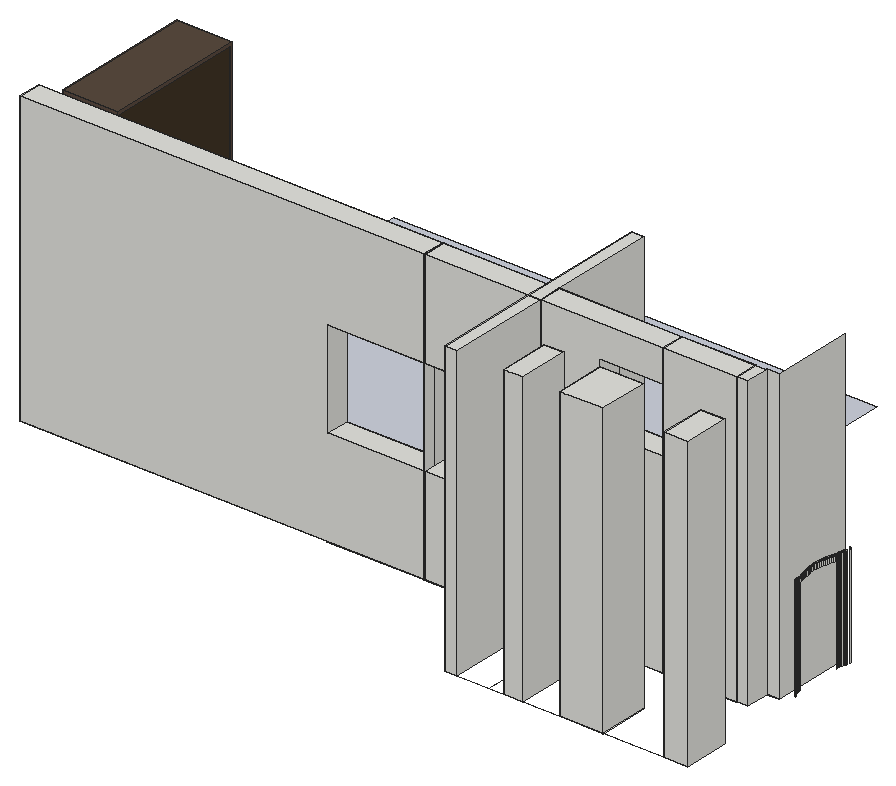
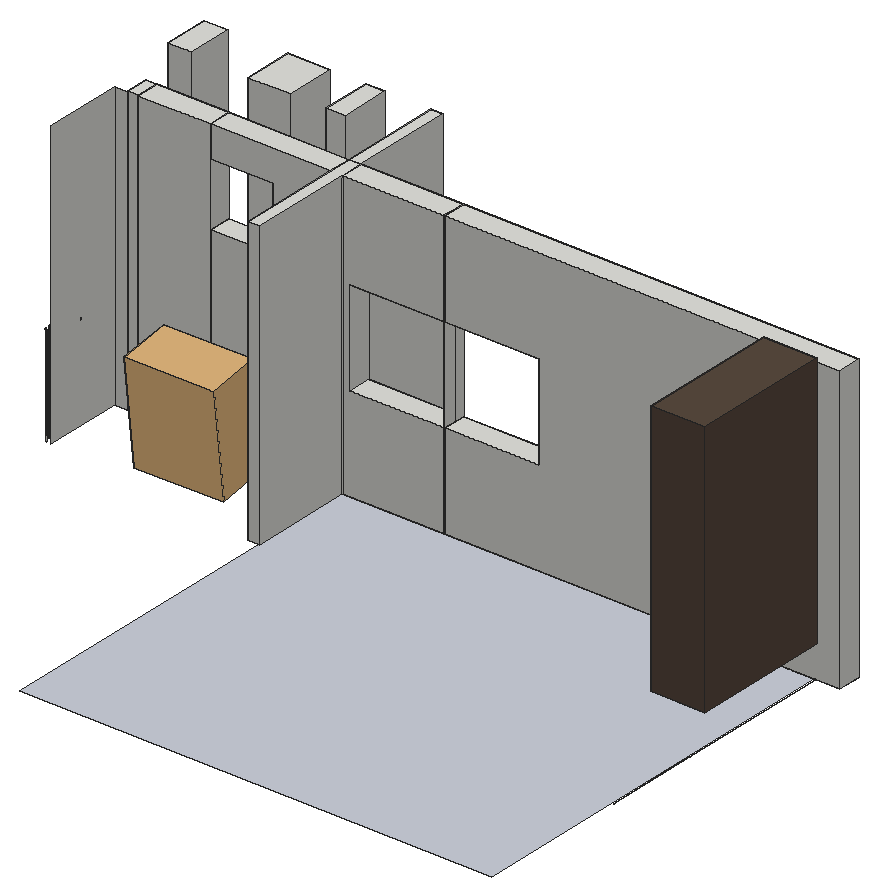
# SketchUp Ruby script. Lengths in inches.
U = 1.inch
M = Sketchup.active_model
def pt(a) = Geom::Point3d.new(a.map { |v| v * U })
def face(e, loops, mat)
  f = e.add_face(loops[0].map { |a| pt(a) })
  loops[1..].each { |l| e.add_face(l.map { |a| pt(a) }).erase! }
  f.material = f.back_material = mat if mat
  f
end
# faces: each face lists its corners as indices into pts; further lists are holes
def faces(e, pts, list, mat = nil) = list.each { |f| face(e, (f[0].is_a?(Array) ? f : [f]).map { |l| l.map { |i| pts[i] } }, mat) }
# xy, xz, yz: faces in a plane at the given z, y or x. An outline is a flat list of corners, or four numbers for a rectangle; further outlines are holes
def ring(l) = l.size == 4 ? [[l[0], l[1]], [l[2], l[1]], [l[2], l[3]], [l[0], l[3]]] : l.each_slice(2).to_a
def flat(e, list, mat, &to3) = list.each { |f| face(e, (f[0].is_a?(Array) ? f : [f]).map { |l| ring(l).map { |u, v| to3.(u, v) } }, mat) }
def xy(e, z, list, mat = nil) = flat(e, list, mat) { |x, y| [x, y, z] }
def xz(e, y, list, mat = nil) = flat(e, list, mat) { |x, z| [x, y, z] }
def yz(e, x, list, mat = nil) = flat(e, list, mat) { |y, z| [x, y, z] }
def lines(e, pts, list) = list.each { |a, b| e.add_line(pt(pts[a]), pt(pts[b])) }
# prism: a flat outline (further loops are holes) pulled along v
def prism(e, loops, v, mat = nil)
  f = face(e, loops, mat); d = Geom::Vector3d.new(v.map { |x| x * U })
  f.pushpull(f.normal.samedirection?(d) ? d.length : -d.length)
end
def box(e, o, s, mat = nil) = prism(e, [[o, [o[0] + s[0], o[1], o[2]], [o[0] + s[0], o[1] + s[1], o[2]], [o[0], o[1] + s[1], o[2]]]], [0, 0, s[2]], mat)
def at(x, y, z, deg = 0) = Geom::Transformation.translation(pt([x, y, z])) * Geom::Transformation.rotation(ORIGIN, Z_AXIS, deg.degrees)
def axes(o, x, y, z) = Geom::Transformation.new([*x, 0, *y, 0, *z, 0, *pt(o).to_a, 1])
def part(name) = M.definitions.add(name)
# library, detail: a bought-in or finely detailed component or shape, given as its bounding box
def library(name, o, s) = part(name).tap { |d| box(d.entities, o, s) }
def detail(e, o, s) = box(e.add_group.entities, o, s)
def put(e, d, t, mat = nil) = e.add_instance(d, t).tap { |i| i.material = mat if mat }
def group(e, t, mat = nil) = e.add_group.tap { |g| g.transformation = t; g.material = mat if mat }.entities
root = M.entities
M.materials.add("[Color A02]").color = [65, 53, 38]
M.materials.add("[Marble Carrara Floor Tile]").color = [204, 208, 219]
M.materials.add("[Wood Veneer 01]").color = [89, 74, 63]
c1 = library("Group\#73",[0,0,0],[33.36,19.5,40.28])
c2 = part("Component\#1")
xy(c2.entities,0,[[0,0,0,29.53,70.87,29.53,70.87,0,69.88,0,69.88,0.98,0.98,0.98,0.98,0]],"[Wood Veneer 01]")
xy(c2.entities,77.76,[[0.98,0,69.88,0.98]])
xy(c2.entities,78.74,[[0,0,70.87,29.53]],"[Wood Veneer 01]")
xz(c2.entities,0,[[0,0,0.98,0,0.98,77.76,69.88,77.76,69.88,0,70.87,0,70.87,78.74,0,78.74]],"[Wood Veneer 01]")
xz(c2.entities,0.98,[[0.98,0.98,69.88,77.76]])
xz(c2.entities,0.98,[[0.98,0,69.88,0.98]],"[Wood Veneer 01]")
xz(c2.entities,29.53,[[0,0,70.87,78.74]],"[Wood Veneer 01]")
yz(c2.entities,0,[[0,0,29.53,78.74]],"[Wood Veneer 01]")
yz(c2.entities,0.98,[[0,0,0.98,0.98],[0,0.98,0.98,77.76]],"[Wood Veneer 01]")
yz(c2.entities,69.88,[[0,0,0.98,0.98],[0,0.98,0.98,77.76]],"[Wood Veneer 01]")
yz(c2.entities,70.87,[[0,0,29.53,78.74]],"[Wood Veneer 01]")
xy(root,0,[[283.6875,0,299.97,0.09],[299.73,0.09,299.97,18.91],[166.56,38.625,202.24,38.86],[202.24,38.625,202.56,38.86],[202.56,38.625,238.24,38.86],
  [282.63,38.625,291.08,38.86],[291.08,38.625,318.375,38.86],[318.375,38.625,318.63,38.86],[267.52,38.86,291.08,47.625],[291.08,38.86,318.375,47.625],
  [318.375,38.86,318.63,47.625],[62.1,45.23,241,45.23,241,47.86,83.3,47.86,83.3,47.83,62.1,47.83],[245.5,47.625,291.08,47.86],[291.08,47.625,318.375,47.86],[318.375,47.625,322.5,47.86],
  [322.5,47.625,327,47.86],[61.56,47.83,62.1,47.86],[62.1,47.83,72.0625,47.86],[61.5,47.86,61.56,107.65],[61.5,107.65,61.56,107.65,61.56,113,61.53,113,61.53,143.65,61.5,143.65]])
xy(root,0,[[62.1,47.86,241,200.36]],"[Marble Carrara Floor Tile]")
xz(root,47.86,[[322.5,0,327,108]])
yz(root,327,[[47.86,0,78.05,108]])
yz(root,328.72,[[54.53,0,54.73,37.7],[54.73,0,54.93,37.7],[72.76,0,72.96,37.7],[72.96,0,73.15,37.7],[54.53,37.7,54.73,37.8],
  [54.73,37.7,54.93,37.8],[72.76,37.7,72.96,37.8],[72.96,37.7,73.15,37.8]])
p = [[329.87,52.03,0],[329.87,52.03,37.7],[329.75,52.0625,37.7],[329.75,52.0625,0],[329.63,52.11,0],[329.63,52.11,37.7],
  [329.51,52.16,37.7],[329.51,52.16,0],[329.4,52.23,0],[329.4,52.23,37.7],[329.3,52.31,37.7],[329.3,52.31,0],
  [329.21,52.4,37.7],[329.21,52.4,0],[329.13,52.49,37.7],[329.13,52.49,0],[329.06,52.6,37.7],[329.06,52.6,0],
  [329,52.71,37.7],[329,52.71,0],[328.95,52.83,37.7],[328.95,52.83,0],[328.91,52.96,37.7],[328.91,52.96,0],
  [328.875,53.15,37.7],[328.875,53.15,0],[328.84,53.35,37.7],[328.84,53.35,0],[328.81,53.54,37.7],[328.81,53.54,0],
  [328.78,53.74,37.7],[328.78,53.74,0],[328.76,53.9375,37.7],[328.76,53.9375,0],[328.74,54.14,37.7],[328.74,54.14,0],
  [328.73,54.33,37.7],[328.73,54.33,0],[328.72,54.53,37.7],[328.72,54.53,0],[328.72,54.93,0],[328.72,54.93,37.7],
  [328.73,55.13,37.7],[328.73,55.13,0],[328.74,55.33,37.7],[328.74,55.33,35.76],[328.74,55.33,0],[328.74,72.36,35.76],
  [328.74,72.36,37.7],[328.73,72.56,37.7],[328.73,72.56,0],[328.74,72.36,0],[328.72,72.76,37.7],[328.72,72.76,0],
  [328.72,73.15,0],[328.72,73.15,37.7],[328.73,73.35,37.7],[328.73,73.35,0],[328.74,73.55,37.7],[328.74,73.55,0],
  [328.76,73.75,37.7],[328.76,73.75,0],[328.78,73.95,37.7],[328.78,73.95,0],[328.81,74.14,37.7],[328.81,74.14,0],
  [328.84,74.34,37.7],[328.84,74.34,0],[328.875,74.53,37.7],[328.875,74.53,0],[328.91,74.73,37.7],[328.91,74.73,0],
  [328.95,74.85,37.7],[328.95,74.85,0],[329,74.97,37.7],[329,74.97,0],[329.06,75.08,37.7],[329.06,75.08,0],
  [329.13,75.19,37.7],[329.13,75.19,0],[329.21,75.29,37.7],[329.21,75.29,0],[329.3,75.38,37.7],[329.3,75.38,0],
  [329.4,75.46,37.7],[329.4,75.46,0],[329.51,75.52,37.7],[329.51,75.52,0],[329.63,75.58,37.7],[329.63,75.58,0],
  [329.75,75.625,37.7],[329.75,75.625,0],[329.87,75.65,37.7],[329.87,75.65,0],[329.75,77.3125,0],[329.75,77.3125,37.7],
  [329.63,77.36,37.7],[329.63,77.36,0],[329.87,77.28,0],[329.87,77.28,37.7],[329.51,77.41,0],[329.51,77.41,37.7],
  [329.4,77.48,37.7],[329.4,77.48,0],[329.3,77.56,37.7],[329.3,77.56,0],[329.21,77.65,0],[329.21,77.65,37.7],
  [329.13,77.74,37.7],[329.13,77.74,0],[328.52,56.02,37.7],[328.52,56.02,35.76],[328.31,56.71,37.7],[328.31,56.71,35.76],
  [328.12,57.41,37.7],[328.12,57.41,35.76],[327.94,58.12,37.7],[327.94,58.12,35.76],[327.78,58.82,37.7],[327.78,58.82,35.76],
  [327.625,59.53,37.7],[327.625,59.53,35.76],[327.49,60.25,37.7],[327.49,60.25,35.76],[327.36,60.96,37.7],[327.36,60.96,35.76],
  [327.25,61.68,37.7],[327.25,61.68,35.76],[327.15,62.4,37.7],[327.15,62.4,35.76],[327.07,63.12,37.7],[327.07,63.12,35.76],
  [327,63.84,37.7],[327,63.84,35.76],[327.07,64.57,37.7],[327.07,64.57,35.76],[327.15,65.29,37.7],[327.15,65.29,35.76],
  [327.25,66.01,37.7],[327.25,66.01,35.76],[327.36,66.72,37.7],[327.36,66.72,35.76],[327.49,67.4375,37.7],[327.49,67.4375,35.76],
  [327.625,68.15,37.7],[327.625,68.15,35.76],[327.78,68.86,37.7],[327.78,68.86,35.76],[327.94,69.57,37.7],[327.94,69.57,35.76],
  [328.12,70.27,37.7],[328.12,70.27,35.76],[328.31,70.97,37.7],[328.31,70.97,35.76],[328.52,71.67,37.7],[328.52,71.67,35.76],
  [329.875,52.04,37.8],[329.75,52.07,37.8],[329.63,52.11,37.8],[329.51,52.16,37.8],[329.4,52.23,37.8],[329.3,52.31,37.8],
  [329.21,52.4,37.8],[329.13,52.5,37.8],[329.06,52.6,37.8],[329,52.72,37.8],[328.95,52.84,37.8],[328.92,52.96,37.8],
  [328.875,53.15,37.8],[328.84,53.35,37.8],[328.81,53.54,37.8],[328.78,53.74,37.8],[328.76,53.9375,37.8],[328.74,54.14,37.8],
  [328.73,54.33,37.8],[328.72,54.53,37.8],[328.72,54.93,37.8],[328.73,55.13,37.8],[328.74,55.33,37.8],[328.52,56.02,37.8],
  [328.32,56.72,37.8],[328.125,57.42,37.8],[327.95,58.12,37.8],[327.78,58.83,37.8],[327.63,59.54,37.8],[327.49,60.25,37.8],
  [327.37,60.96,37.8],[327.25,61.68,37.8],[327.16,62.4,37.8],[327.07,63.12,37.8],[327,63.84,37.8],[327.07,64.57,37.8],
  [327.16,65.29,37.8],[327.25,66.01,37.8],[327.37,66.72,37.8],[327.49,67.4375,37.8],[327.63,68.15,37.8],[327.78,68.86,37.8],
  [327.95,69.57,37.8],[328.125,70.27,37.8],[328.32,70.97,37.8],[328.52,71.67,37.8],[328.74,72.36,37.8],[328.73,72.56,37.8],
  [328.72,72.76,37.8],[328.72,73.15,37.8],[328.73,73.35,37.8],[328.74,73.55,37.8],[328.76,73.75,37.8],[328.78,73.95,37.8],
  [328.81,74.14,37.8],[328.84,74.34,37.8],[328.875,74.53,37.8],[328.92,74.73,37.8],[328.95,74.85,37.8],[329,74.97,37.8],
  [329.06,75.08,37.8],[329.13,75.1875,37.8],[329.21,75.29,37.8],[329.3,75.375,37.8],[329.4,75.45,37.8],[329.51,75.52,37.8],
  [329.63,75.58,37.8],[329.75,75.62,37.8],[329.875,75.65,37.8],[329.75,77.32,37.8],[329.63,77.36,37.8],[329.875,77.29,37.8],
  [329.51,77.41,37.8],[329.4,77.48,37.8],[329.3,77.56,37.8],[329.21,77.65,37.8],[329.875,52.05,37.89],[329.75,52.08,37.89],
  [329.63,52.12,37.89],[329.52,52.17,37.89],[329.41,52.24,37.89],[329.3125,52.32,37.89],[329.22,52.41,37.89],[329.14,52.5,37.89],
  [329.07,52.61,37.89],[329.01,52.72,37.89],[328.96,52.84,37.89],[328.93,52.96,37.89],[328.89,53.15,37.89],[328.85,53.35,37.89],
  [328.82,53.55,37.89],[328.79,53.74,37.89],[328.77,53.9375,37.89],[328.76,54.14,37.89],[328.74,54.33,37.89],[328.74,54.53,37.89],
  [328.72,54.73,37.8],[328.73,54.73,37.89],[328.74,54.93,37.89],[328.74,55.13,37.89],[328.76,55.33,37.89],[328.54,56.02,37.89],
  [328.33,56.72,37.89],[328.14,57.42,37.89],[327.96,58.12,37.89],[327.79,58.83,37.89],[327.64,59.54,37.89],[327.5,60.25,37.89],
  [327.375,60.96,37.89],[327.27,61.68,37.89],[327.17,62.4,37.89],[327.08,63.12,37.89],[327.01,63.84,37.89],[327.08,64.5625,37.89],
  [327.17,65.28,37.89],[327.27,66,37.89],[327.375,66.72,37.89],[327.5,67.4375,37.89],[327.64,68.15,37.89],[327.79,68.86,37.89],
  [327.96,69.5625,37.89],[328.14,70.27,37.89],[328.33,70.97,37.89],[328.54,71.66,37.89],[328.76,72.36,37.89],[328.74,72.56,37.89],
  [328.74,72.76,37.89],[328.72,72.96,37.8],[328.73,72.96,37.89],[328.74,73.15,37.89],[328.74,73.35,37.89],[328.76,73.55,37.89],
  [328.77,73.75,37.89],[328.79,73.94,37.89],[328.82,74.14,37.89],[328.85,74.34,37.89],[328.89,74.53,37.89],[328.93,74.72,37.89],
  [328.96,74.85,37.89],[329.01,74.96,37.89],[329.07,75.08,37.89],[329.14,75.18,37.89],[329.22,75.28,37.89],[329.3125,75.37,37.89],
  [329.41,75.44,37.89],[329.52,75.51,37.89],[329.63,75.57,37.89],[329.75,75.61,37.89],[329.875,75.64,37.89],[329.75,77.33,37.89],
  [329.63,77.37,37.89],[329.875,77.3,37.89],[329.52,77.42,37.89],[329.41,77.49,37.89],[329.3125,77.57,37.89],[329.22,77.66,37.89],
  [329.64,52.14,37.99],[329.53,52.19,37.99],[329.76,52.09,37.99],[329.42,52.26,37.99],[329.32,52.33,37.99],[329.23,52.42,37.99],
  [329.15,52.51,37.99],[329.08,52.62,37.99],[329.03,52.73,37.99],[328.98,52.84,37.99],[328.95,52.97,37.99],[328.91,53.16,37.99],
  [328.87,53.35,37.99],[328.84,53.55,37.99],[328.8125,53.74,37.99],[328.79,53.94,37.99],[328.77,54.14,37.99],[328.76,54.34,37.99],
  [328.75,54.53,37.99],[328.75,54.73,37.99],[328.75,54.93,37.99],[328.76,55.125,37.99],[328.77,55.33,37.99],[328.55,56.03,37.99],
  [328.35,56.72,37.99],[328.15,57.42,37.99],[327.98,58.125,37.99],[327.81,58.83,37.99],[327.66,59.54,37.99],[327.52,60.25,37.99],
  [327.39,60.97,37.99],[327.28,61.68,37.99],[327.1875,62.4,37.99],[327.1,63.125,37.99],[327.03,63.84,37.99],[327.1,64.5625,37.99],
  [327.1875,65.28,37.99],[327.28,66,37.99],[327.39,66.72,37.99],[327.52,67.43,37.99],[327.66,68.14,37.99],[327.81,68.85,37.99],
  [327.98,69.56,37.99],[328.15,70.26,37.99],[328.35,70.96,37.99],[328.55,71.66,37.99],[328.77,72.36,37.99],[328.76,72.56,37.99],
  [328.75,72.76,37.99],[328.75,72.96,37.99],[328.75,73.15,37.99],[328.76,73.35,37.99],[328.77,73.55,37.99],[328.79,73.75,37.99],
  [328.8125,73.94,37.99],[328.84,74.14,37.99],[328.87,74.33,37.99],[328.91,74.53,37.99],[328.95,74.72,37.99],[328.98,74.84,37.99],
  [329.03,74.96,37.99],[329.08,75.07,37.99],[329.15,75.17,37.99],[329.23,75.27,37.99],[329.32,75.35,37.99],[329.42,75.43,37.99],
  [329.53,75.5,37.99],[329.64,75.55,37.99],[329.76,75.59,37.99],[329.88,75.62,37.99],[329.76,77.34,37.99],[329.64,77.39,37.99],
  [329.53,77.44,37.99],[329.42,77.51,37.99],[329.32,77.58,37.99],[329.23,77.67,37.99],[329.65,52.16,38.08],[329.54,52.21,38.08],
  [329.77,52.12,38.08],[329.4375,52.28,38.08],[329.34,52.35,38.08],[329.25,52.4375,38.08],[329.17,52.53,38.08],[329.11,52.63,38.08],
  [329.05,52.74,38.08],[329,52.85,38.08],[328.97,52.97,38.08],[328.93,53.16,38.08],[328.9,53.36,38.08],[328.86,53.55,38.08],
  [328.84,53.75,38.08],[328.82,53.94,38.08],[328.8,54.14,38.08],[328.79,54.34,38.08],[328.78,54.53,38.08],[328.78,54.73,38.08],
  [328.78,54.93,38.08],[328.79,55.125,38.08],[328.8,55.33,38.08],[328.58,56.04,38.08],[328.37,56.73,38.08],[328.18,57.43,38.08],
  [328,58.13,38.08],[327.84,58.84,38.08],[327.68,59.55,38.08],[327.54,60.26,38.08],[327.42,60.97,38.08],[327.31,61.6875,38.08],
  [327.21,62.41,38.08],[327.13,63.125,38.08],[327.06,63.84,38.08],[327.13,64.56,38.08],[327.21,65.28,38.08],[327.31,66,38.08],
  [327.42,66.71,38.08],[327.54,67.43,38.08],[327.68,68.14,38.08],[327.84,68.85,38.08],[328,69.55,38.08],[328.18,70.26,38.08],
  [328.37,70.96,38.08],[328.58,71.65,38.08],[328.8,72.35,38.08],[328.79,72.5625,38.08],[328.78,72.76,38.08],[328.78,72.96,38.08],
  [328.78,73.15,38.08],[328.79,73.35,38.08],[328.8,73.55,38.08],[328.82,73.74,38.08],[328.84,73.9375,38.08],[328.86,74.13,38.08],
  [328.9,74.33,38.08],[328.93,74.52,38.08],[328.97,74.71,38.08],[329,74.83,38.08],[329.05,74.95,38.08],[329.11,75.05,38.08],
  [329.17,75.16,38.08],[329.25,75.25,38.08],[329.34,75.33,38.08],[329.4375,75.41,38.08],[329.54,75.47,38.08],[329.65,75.53,38.08],
  [329.77,75.57,38.08],[329.77,77.37,38.08],[329.65,77.41,38.08],[329.54,77.46,38.08],[329.4375,77.53,38.08],[329.34,77.6,38.08],
  [329.25,77.6875,38.08],[329.77,52.15,38.17],[329.66,52.19,38.17],[329.56,52.24,38.17],[329.46,52.3,38.17],[329.36,52.38,38.17],
  [329.28,52.46,38.17],[329.2,52.55,38.17],[329.13,52.65,38.17],[329.08,52.75,38.17],[329.04,52.86,38.17],[329,52.98,38.17],
  [328.96,53.17,38.17],[328.93,53.36,38.17],[328.9,53.56,38.17],[328.87,53.75,38.17],[328.85,53.95,38.17],[328.83,54.14,38.17],
  [328.82,54.34,38.17],[328.8125,54.53,38.17],[328.8125,54.73,38.17],[328.8125,54.93,38.17],[328.82,55.125,38.17],[328.83,55.34,38.17],
  [328.61,56.05,38.17],[328.4,56.74,38.17],[328.21,57.4375,38.17],[328.03,58.14,38.17],[327.87,58.84,38.17],[327.72,59.55,38.17],
  [327.58,60.26,38.17],[327.45,60.98,38.17],[327.34,61.69,38.17],[327.24,62.41,38.17],[327.16,63.13,38.17],[327.09,63.84,38.17],
  [327.16,64.56,38.17],[327.24,65.28,38.17],[327.34,65.99,38.17],[327.45,66.71,38.17],[327.58,67.42,38.17],[327.72,68.13,38.17],
  [327.87,68.84,38.17],[328.03,69.55,38.17],[328.21,70.25,38.17],[328.4,70.95,38.17],[328.61,71.64,38.17],[328.83,72.35,38.17],
  [328.82,72.5625,38.17],[328.8125,72.76,38.17],[328.8125,72.96,38.17],[328.8125,73.15,38.17],[328.82,73.35,38.17],[328.83,73.54,38.17],
  [328.85,73.74,38.17],[328.87,73.93,38.17],[328.9,74.13,38.17],[328.93,74.32,38.17],[328.96,74.52,38.17],[329,74.71,38.17],
  [329.04,74.82,38.17],[329.08,74.93,38.17],[329.13,75.04,38.17],[329.2,75.14,38.17],[329.28,75.23,38.17],[329.36,75.31,38.17],
  [329.46,75.38,38.17],[329.56,75.44,38.17],[329.66,75.5,38.17],[329.77,75.54,38.17],[329.66,77.44,38.17],[329.56,77.49,38.17],
  [329.77,77.4,38.17],[329.46,77.55,38.17],[329.36,77.63,38.17],[329.28,77.71,38.17],[329.68,52.23,38.26],[329.58,52.28,38.26],
  [329.23,52.57,38.26],[329.17,52.67,38.26],[329.12,52.77,38.26],[329.07,52.875,38.26],[327.28,62.42,38.26],[327.2,63.13,38.26],
  [327.38,65.99,38.26],[327.49,66.7,38.26],[327.62,67.41,38.26],[327.75,68.125,38.26],[327.91,68.83,38.26],[328.07,69.54,38.26],
  [328.25,70.24,38.26],[328.44,70.94,38.26],[328.65,71.63,38.26],[328.875,72.34,38.26],[328.86,72.5625,38.26],[328.85,72.76,38.26],
  [328.85,72.96,38.26],[328.85,73.15,38.26],[328.86,73.35,38.26],[328.87,73.54,38.26],[328.89,73.74,38.26],[329.04,74.7,38.26],
  [329.07,74.81,38.26],[329.12,74.92,38.26],[329.39,75.28,38.26],[329.48,75.35,38.26],[329.68,75.46,38.26],[329.79,75.5,38.26],
  [322.42,26.12,0],[322.42,17.12,0],[257.39,0.09,0],[257.39,32.63,0],[282.84,32.63,0],[282.84,38.625,0],
  [166.56,47.625,0],[202.24,47.625,0],[238.24,43.125,0],[202.56,43.125,0],[72.79,47.86,0],[72.79,47.83,0],
  [282.84,38.77,0],[202.56,47.625,0],[238.24,47.625,0],[245.5,0.09,0],[262.84,0.09,0],[283.6875,0.09,0],
  [270.15,0.09,0],[322.42,0.09,0],[299.97,0.09,0],[166.56,43.125,0],[166.56,45.23,0],[202.24,43.125,0],
  [166.56,38.86,0],[52.5,38.86,0],[52.5,47.625,0],[245.5,38.86,0],[238.24,38.86,0]]
faces(root,p,[[0,1,2,3],[4,5,6,7],[3,2,5,4],[8,9,10,11],[7,6,9,8],[11,10,12,13],[13,12,14,15],[15,14,16,17],
  [17,16,18,19],[19,18,20,21],[21,20,22,23],[23,22,24,25],[25,24,26,27],[27,26,28,29],[29,28,30,31],[31,30,32,33],
  [33,32,34,35],[35,34,36,37],[37,36,38,39],[40,41,42,43],[43,42,44,45,46],[47,48,49,50,51],[50,49,52,53],[54,55,56,57],
  [57,56,58,59],[59,58,60,61],[61,60,62,63],[63,62,64,65],[65,64,66,67],[67,66,68,69],[69,68,70,71],[71,70,72,73],
  [73,72,74,75],[75,74,76,77],[77,76,78,79],[79,78,80,81],[81,80,82,83],[83,82,84,85],[85,84,86,87],[87,86,88,89],
  [89,88,90,91],[91,90,92,93],[94,95,96,97],[98,99,95,94],[100,101,102,103],[97,96,101,100],[103,102,104,105],[106,107,108,109],
  [105,104,107,106],[45,44,110,111],[111,110,112,113],[113,112,114,115],[115,114,116,117],[117,116,118,119],[119,118,120,121],[121,120,122,123],
  [123,122,124,125],[125,124,126,127],[127,126,128,129],[129,128,130,131],[131,130,132,133],[133,132,134,135],[135,134,136,137],[137,136,138,139],
  [139,138,140,141],[141,140,142,143],[143,142,144,145],[145,144,146,147],[147,146,148,149],[149,148,150,151],[151,150,152,153],[153,152,154,155],
  [155,154,48,47],[156,1,2,157],[158,5,6,159],[157,2,5,158],[160,9,10,161],[159,6,9,160],[161,10,12,162],[162,12,14,163],
  [163,14,16,164],[164,16,18,165],[165,18,20,166],[166,20,22,167],[167,22,24,168],[168,24,26,169],[169,26,28,170],[170,28,30,171],
  [171,30,32,172],[172,32,34,173],[173,34,36,174],[174,36,38,175],[176,41,42,177],[177,42,44,178],[178,44,110,179],[179,110,112,180],
  [180,112,114,181],[181,114,116,182],[182,116,118,183],[183,118,120,184],[184,120,122,185],[185,122,124,186],[186,124,126,187],[187,126,128,188],
  [188,128,130,189],[189,130,132,190],[190,132,134,191],[191,134,136,192],[192,136,138,193],[193,138,140,194],[194,140,142,195],[195,142,144,196],
  [196,144,146,197],[197,146,148,198],[198,148,150,199],[199,150,152,200],[200,152,154,201],[201,154,48,202],[202,48,49,203],[203,49,52,204],
  [205,55,56,206],[206,56,58,207],[207,58,60,208],[208,60,62,209],[209,62,64,210],[210,64,66,211],[211,66,68,212],[212,68,70,213],
  [213,70,72,214],[214,72,74,215],[215,74,76,216],[216,76,78,217],[217,78,80,218],[218,80,82,219],[219,82,84,220],[220,84,86,221],
  [221,86,88,222],[222,88,90,223],[223,90,92,224],[225,95,96,226],[227,99,95,225],[228,101,102,229],[226,96,101,228],[229,102,104,230],
  [230,104,107,231],[232,156,157,233],[234,158,159,235],[233,157,158,234],[236,160,161,237],[235,159,160,236],[237,161,162,238],[238,162,163,239],
  [239,163,164,240],[240,164,165,241],[241,165,166,242],[242,166,167,243],[243,167,168,244],[244,168,169,245],[245,169,170,246],[246,170,171,247],
  [247,171,172,248],[248,172,173,249],[249,173,174,250],[250,174,175,251],[251,175,252,253],[253,252,176,254],[254,176,177,255],[255,177,178,256],
  [256,178,179,257],[257,179,180,258],[258,180,181,259],[259,181,182,260],[260,182,183,261],[261,183,184,262],[262,184,185,263],[263,185,186,264],
  [264,186,187,265],[265,187,188,266],[266,188,189,267],[267,189,190,268],[268,190,191,269],[269,191,192,270],[270,192,193,271],[271,193,194,272],
  [272,194,195,273],[273,195,196,274],[274,196,197,275],[275,197,198,276],[276,198,199,277],[277,199,200,278],[278,200,201,279],[279,201,202,280],
  [280,202,203,281],[281,203,204,282],[282,204,283,284],[284,283,205,285],[285,205,206,286],[286,206,207,287],[287,207,208,288],[288,208,209,289],
  [289,209,210,290],[290,210,211,291],[291,211,212,292],[292,212,213,293],[293,213,214,294],[294,214,215,295],[295,215,216,296],[296,216,217,297],
  [297,217,218,298],[298,218,219,299],[299,219,220,300],[300,220,221,301],[301,221,222,302],[302,222,223,303],[303,223,224,304],[305,225,226,306],
  [307,227,225,305],[308,228,229,309],[306,226,228,308],[309,229,230,310],[310,230,231,311],[312,234,235,313],[314,233,234,312],[315,236,237,316],
  [313,235,236,315],[316,237,238,317],[317,238,239,318],[318,239,240,319],[319,240,241,320],[320,241,242,321],[321,242,243,322],[322,243,244,323],
  [323,244,245,324],[324,245,246,325],[325,246,247,326],[326,247,248,327],[327,248,249,328],[328,249,250,329],[329,250,251,330],[330,251,253,331],
  [331,253,254,332],[332,254,255,333],[333,255,256,334],[334,256,257,335],[335,257,258,336],[336,258,259,337],[337,259,260,338],[338,260,261,339],
  [339,261,262,340],[340,262,263,341],[341,263,264,342],[342,264,265,343],[343,265,266,344],[344,266,267,345],[345,267,268,346],[346,268,269,347],
  [347,269,270,348],[348,270,271,349],[349,271,272,350],[350,272,273,351],[351,273,274,352],[352,274,275,353],[353,275,276,354],[354,276,277,355],
  [355,277,278,356],[356,278,279,357],[357,279,280,358],[358,280,281,359],[359,281,282,360],[360,282,284,361],[361,284,285,362],[362,285,286,363],
  [363,286,287,364],[364,287,288,365],[365,288,289,366],[366,289,290,367],[367,290,291,368],[368,291,292,369],[369,292,293,370],[370,293,294,371],
  [371,294,295,372],[372,295,296,373],[373,296,297,374],[374,297,298,375],[375,298,299,376],[376,299,300,377],[377,300,301,378],[378,301,302,379],
  [379,302,303,380],[380,303,304,381],[382,305,306,383],[384,308,309,385],[383,306,308,384],[385,309,310,386],[386,310,311,387],[388,312,313,389],
  [390,314,312,388],[389,313,315,391],[392,316,317,393],[391,315,316,392],[393,317,318,394],[394,318,319,395],[395,319,320,396],[396,320,321,397],
  [397,321,322,398],[398,322,323,399],[399,323,324,400],[400,324,325,401],[401,325,326,402],[402,326,327,403],[403,327,328,404],[404,328,329,405],
  [405,329,330,406],[406,330,331,407],[407,331,332,408],[408,332,333,409],[409,333,334,410],[410,334,335,411],[411,335,336,412],[412,336,337,413],
  [413,337,338,414],[414,338,339,415],[415,339,340,416],[416,340,341,417],[417,341,342,418],[418,342,343,419],[419,343,344,420],[420,344,345,421],
  [421,345,346,422],[422,346,347,423],[423,347,348,424],[424,348,349,425],[425,349,350,426],[426,350,351,427],[427,351,352,428],[428,352,353,429],
  [429,353,354,430],[430,354,355,431],[431,355,356,432],[432,356,357,433],[433,357,358,434],[434,358,359,435],[435,359,360,436],[436,360,361,437],
  [437,361,362,438],[438,362,363,439],[439,363,364,440],[440,364,365,441],[441,365,366,442],[442,366,367,443],[443,367,368,444],[444,368,369,445],
  [445,369,370,446],[446,370,371,447],[447,371,372,448],[448,372,373,449],[449,373,374,450],[450,374,375,451],[451,375,376,452],[452,376,377,453],
  [453,377,378,454],[454,378,379,455],[455,379,380,456],[457,382,383,458],[459,384,385,460],[458,383,384,459],[460,385,386,461],[461,386,387,462],
  [463,390,388,464],[465,389,391,466],[464,388,389,465],[466,391,392,467],[468,393,394,469],[467,392,393,468],[469,394,395,470],[470,395,396,471],
  [471,396,397,472],[472,397,398,473],[473,398,399,474],[474,399,400,475],[475,400,401,476],[476,401,402,477],[477,402,403,478],[478,403,404,479],
  [479,404,405,480],[480,405,406,481],[481,406,407,482],[482,407,408,483],[483,408,409,484],[484,409,410,485],[485,410,411,486],[486,411,412,487],
  [487,412,413,488],[488,413,414,489],[489,414,415,490],[490,415,416,491],[491,416,417,492],[492,417,418,493],[493,418,419,494],[494,419,420,495],
  [495,420,421,496],[496,421,422,497],[497,422,423,498],[498,423,424,499],[499,424,425,500],[500,425,426,501],[501,426,427,502],[502,427,428,503],
  [503,428,429,504],[504,429,430,505],[505,430,431,506],[506,431,432,507],[507,432,433,508],[508,433,434,509],[509,434,435,510],[510,435,436,511],
  [511,436,437,512],[512,437,438,513],[513,438,439,514],[514,439,440,515],[515,440,441,516],[516,441,442,517],[517,442,443,518],[518,443,444,519],
  [519,444,445,520],[520,445,446,521],[521,446,447,522],[522,447,448,523],[523,448,449,524],[524,449,450,525],[525,450,451,526],[526,451,452,527],
  [527,452,453,528],[528,453,454,529],[529,454,455,530],[530,455,456,531],[532,458,459,533],[534,457,458,532],[535,460,461,536],[533,459,460,535],
  [536,461,462,537],[538,464,465,539],[540,469,470,541],[541,470,471,542],[542,471,472,543],[544,495,496,545],[546,500,501,547],[547,501,502,548],
  [548,502,503,549],[549,503,504,550],[550,504,505,551],[551,505,506,552],[552,506,507,553],[554,508,509,555],[555,509,510,556],[557,511,512,558],
  [559,513,514,560],[561,515,516,562],[563,521,522,564],[564,522,523,565],[566,527,528,567],[568,530,531,569]])
lines(root,p,[[570,571],[572,573],[574,575],[576,577],[578,579],[580,581],[575,582],[583,584],[572,585],[586,572],[587,588],[589,590],
  [573,574],[591,592],[593,591],[594,591],[595,596],[594,595],[592,576],[597,598],[571,589]])
g1 = group(root,at(322.42,0.09,0))
box(g1,[0,0,0],[9,17.03,108])
g2 = group(root,at(262.84,0.09,0))
box(g2,[0,0,0],[7.31,18.82,108])
g3 = group(root,at(283.6875,0.09,0))
box(g3,[0,0,0],[16.04,18.82,108])
g4 = group(root,at(241,0.09,0))
box(g4,[0,0,0],[4.5,38.77,108])
g5 = group(root,at(202.24,38.86,0))
box(g5,[0,0,0],[0.3125,4.27,108])
g6 = group(root,at(52.5,38.86,0))
prism(g6,[[[0,0,0],[149.68,0,0],[149.68,0,36],[114.06,0,36],[114.06,0,72],[149.68,0,72],[149.68,0,108],[0,0,108]]],[0,8.77,0])
g7 = group(root,at(238.24,38.86,0))
prism(g7,[[[-36.0625,0,0],[2.76,0,0],[2.76,0,108],[-36.0625,0,108],[-36.0625,0,72],[0,0,72],[0,0,36],[-36.0625,0,36]]],[0,8.77,0])
g8 = group(root,at(245.5,38.86,0))
prism(g8,[[[0,0,0],[45.52,0,0],[45.52,0,72],[22.02,0,72],[22.02,0,96],[45.58,0,96],[45.58,0,108],[0,0,108]]],[0,8.77,0])
g9 = group(root,at(291.08,38.86,0))
box(g9,[0,0,0],[27.29,8.77,108])
g10 = group(root,at(318.63,38.86,0))
xy(g10,0,[[0,0,3.87,8.77]])
xy(g10,108,[[0,0,3.87,8.77]])
xz(g10,0,[[0,0,3.87,108]])
xz(g10,8.77,[[0,0,3.87,108]])
yz(g10,3.87,[[0,0,8.77,108]])
g11 = group(root,at(202.24,43.125,0))
box(g11,[0,0,0],[0.3125,4.5,108])
g12 = group(root,at(241,38.86,0))
prism(g12,[[[4.5,0,0],[0,0,0],[0,8.77,0],[0,9,0],[0,48.05,0],[4.5,48.05,0],[4.5,9,0]]],[0,0,108])
put(root,c1,axes([300.17,72.5,-1.08],[-0.9997,-0.02334,-0.00774],[0.02213,-0.99123,0.1303],[-0.01071,0.13009,0.99144]))
put(root,c2,axes([81.54,47.625,12.25],[0,0.75,0],[-0.69,0,0],[0,0,1.23]),"[Color A02]")
